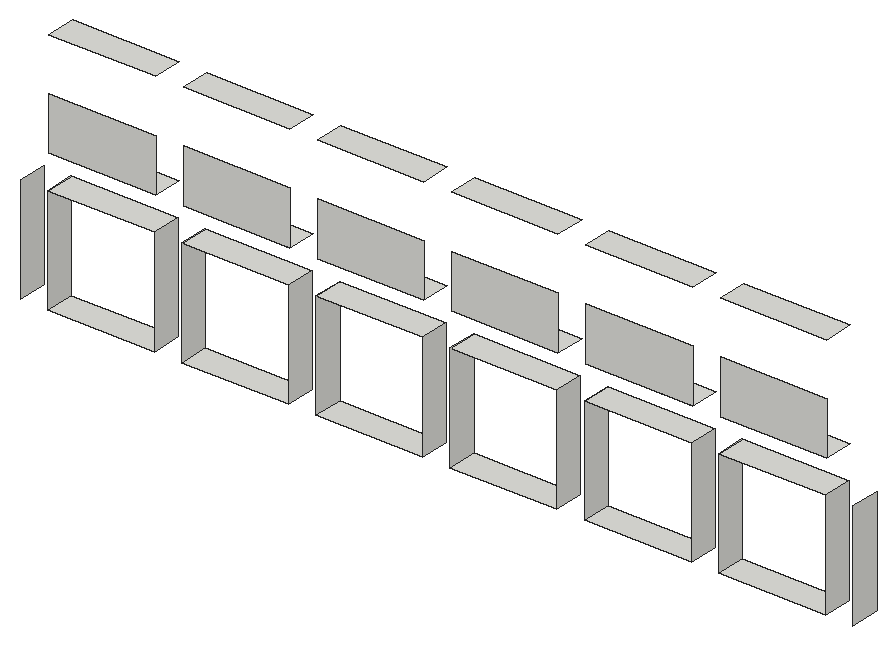
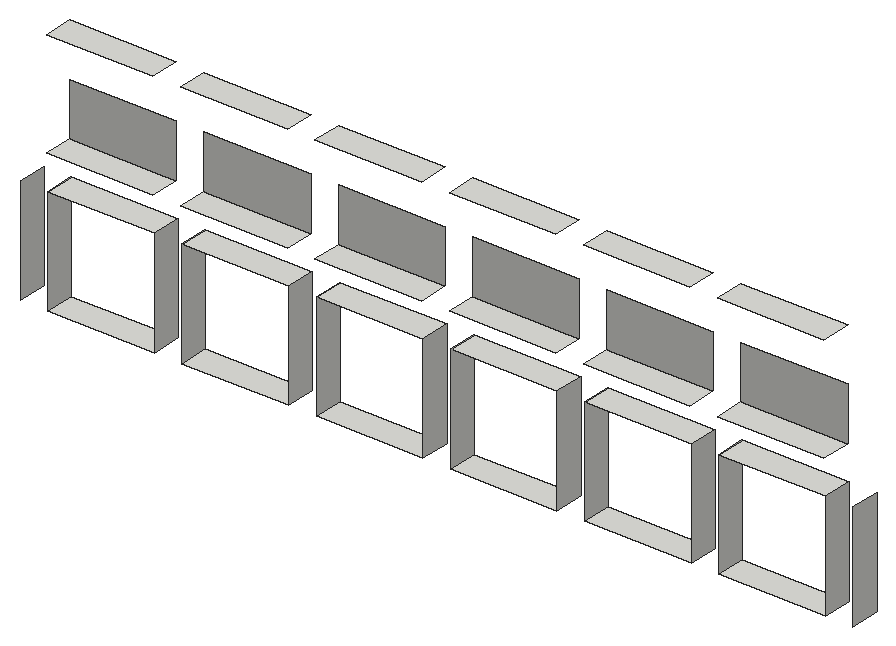
# SketchUp Ruby script. Lengths in inches.
U = 1.inch
M = Sketchup.active_model
def pt(a) = Geom::Point3d.new(a.map { |v| v * U })
def face(e, loops, mat)
  f = e.add_face(loops[0].map { |a| pt(a) })
  loops[1..].each { |l| e.add_face(l.map { |a| pt(a) }).erase! }
  f.material = f.back_material = mat if mat
  f
end
# faces: each face lists its corners as indices into pts; further lists are holes
def faces(e, pts, list, mat = nil) = list.each { |f| face(e, (f[0].is_a?(Array) ? f : [f]).map { |l| l.map { |i| pts[i] } }, mat) }
# xy, xz, yz: faces in a plane at the given z, y or x. An outline is a flat list of corners, or four numbers for a rectangle; further outlines are holes
def ring(l) = l.size == 4 ? [[l[0], l[1]], [l[2], l[1]], [l[2], l[3]], [l[0], l[3]]] : l.each_slice(2).to_a
def flat(e, list, mat, &to3) = list.each { |f| face(e, (f[0].is_a?(Array) ? f : [f]).map { |l| ring(l).map { |u, v| to3.(u, v) } }, mat) }
def xy(e, z, list, mat = nil) = flat(e, list, mat) { |x, y| [x, y, z] }
def xz(e, y, list, mat = nil) = flat(e, list, mat) { |x, z| [x, y, z] }
def yz(e, x, list, mat = nil) = flat(e, list, mat) { |y, z| [x, y, z] }
def lines(e, pts, list) = list.each { |a, b| e.add_line(pt(pts[a]), pt(pts[b])) }
# prism: a flat outline (further loops are holes) pulled along v
def prism(e, loops, v, mat = nil)
  f = face(e, loops, mat); d = Geom::Vector3d.new(v.map { |x| x * U })
  f.pushpull(f.normal.samedirection?(d) ? d.length : -d.length)
end
def box(e, o, s, mat = nil) = prism(e, [[o, [o[0] + s[0], o[1], o[2]], [o[0] + s[0], o[1] + s[1], o[2]], [o[0], o[1] + s[1], o[2]]]], [0, 0, s[2]], mat)
def at(x, y, z, deg = 0) = Geom::Transformation.translation(pt([x, y, z])) * Geom::Transformation.rotation(ORIGIN, Z_AXIS, deg.degrees)
def axes(o, x, y, z) = Geom::Transformation.new([*x, 0, *y, 0, *z, 0, *pt(o).to_a, 1])
def part(name) = M.definitions.add(name)
# library, detail: a bought-in or finely detailed component or shape, given as its bounding box
def library(name, o, s) = part(name).tap { |d| box(d.entities, o, s) }
def detail(e, o, s) = box(e.add_group.entities, o, s)
def put(e, d, t, mat = nil) = e.add_instance(d, t).tap { |i| i.material = mat if mat }
def group(e, t, mat = nil) = e.add_group.tap { |g| g.transformation = t; g.material = mat if mat }.entities
root = M.entities
xy(root,259.68,[[1330.85,480.14,1333.16,480.77],[1333.76,480.14,1336.07,480.77],[1336.67,480.14,1338.98,480.77],[1339.58,480.14,1341.89,480.77],[1342.49,480.14,1344.81,480.77],
  [1345.41,480.14,1347.72,480.77]])
xy(root,262,[[1330.85,480.14,1333.16,480.77],[1333.76,480.14,1336.07,480.77],[1336.67,480.14,1338.98,480.77],[1339.58,480.14,1341.89,480.77],[1342.49,480.14,1344.81,480.77],
  [1345.41,480.14,1347.72,480.77]])
xy(root,262.73,[[1330.875,480.14,1333.1875,480.77],[1333.79,480.14,1336.1,480.77],[1336.7,480.14,1339.01,480.77],[1339.61,480.14,1341.92,480.77],[1342.52,480.14,1344.84,480.77],
  [1345.44,480.14,1347.75,480.77]])
xy(root,265.04,[[1330.875,480.14,1333.1875,480.77],[1333.79,480.14,1336.1,480.77],[1336.7,480.14,1339.01,480.77],[1339.61,480.14,1341.92,480.77],[1342.52,480.14,1344.84,480.77],
  [1345.44,480.14,1347.75,480.77]])
xz(root,480.14,[[1330.875,262.73,1333.1875,263.89],[1333.79,262.73,1336.1,263.89],[1336.7,262.73,1339.01,263.89],[1339.61,262.73,1341.92,263.89],[1342.52,262.73,1344.84,263.89],
  [1345.44,262.73,1347.75,263.89]])
yz(root,1330.25,[[480.14,259.68,480.77,262]])
yz(root,1330.85,[[480.14,259.68,480.77,262]])
yz(root,1333.16,[[480.14,259.68,480.77,262]])
yz(root,1333.76,[[480.14,259.68,480.77,262]])
yz(root,1336.07,[[480.14,259.68,480.77,262]])
yz(root,1336.67,[[480.14,259.68,480.77,262]])
yz(root,1338.98,[[480.14,259.68,480.77,262]])
yz(root,1339.58,[[480.14,259.68,480.77,262]])
yz(root,1341.89,[[480.14,259.68,480.77,262]])
yz(root,1342.49,[[480.14,259.68,480.77,262]])
yz(root,1344.81,[[480.14,259.68,480.77,262]])
yz(root,1345.41,[[480.14,259.68,480.77,262]])
yz(root,1347.72,[[480.14,259.68,480.77,262]])
yz(root,1348.32,[[480.14,259.68,480.77,262]])
